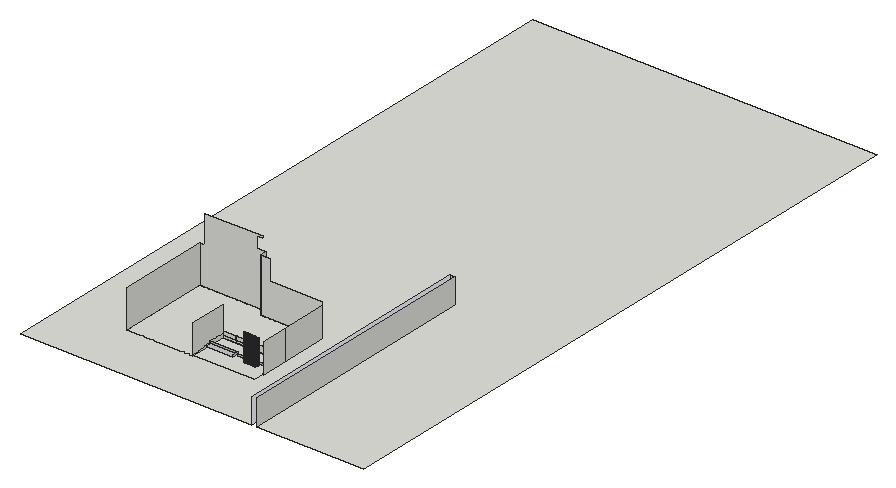
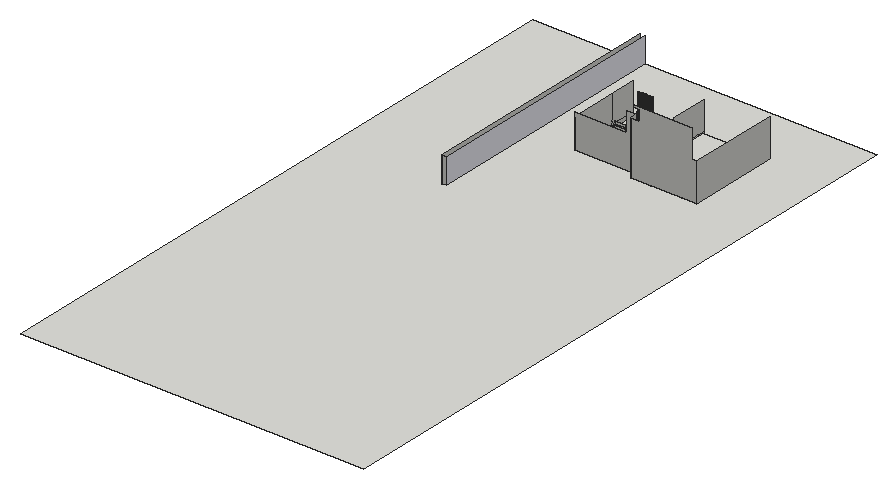
# SketchUp Ruby script. Lengths in inches.
U = 1.inch
M = Sketchup.active_model
def pt(a) = Geom::Point3d.new(a.map { |v| v * U })
def face(e, loops, mat)
  f = e.add_face(loops[0].map { |a| pt(a) })
  loops[1..].each { |l| e.add_face(l.map { |a| pt(a) }).erase! }
  f.material = f.back_material = mat if mat
  f
end
# faces: each face lists its corners as indices into pts; further lists are holes
def faces(e, pts, list, mat = nil) = list.each { |f| face(e, (f[0].is_a?(Array) ? f : [f]).map { |l| l.map { |i| pts[i] } }, mat) }
# xy, xz, yz: faces in a plane at the given z, y or x. An outline is a flat list of corners, or four numbers for a rectangle; further outlines are holes
def ring(l) = l.size == 4 ? [[l[0], l[1]], [l[2], l[1]], [l[2], l[3]], [l[0], l[3]]] : l.each_slice(2).to_a
def flat(e, list, mat, &to3) = list.each { |f| face(e, (f[0].is_a?(Array) ? f : [f]).map { |l| ring(l).map { |u, v| to3.(u, v) } }, mat) }
def xy(e, z, list, mat = nil) = flat(e, list, mat) { |x, y| [x, y, z] }
def xz(e, y, list, mat = nil) = flat(e, list, mat) { |x, z| [x, y, z] }
def yz(e, x, list, mat = nil) = flat(e, list, mat) { |y, z| [x, y, z] }
def lines(e, pts, list) = list.each { |a, b| e.add_line(pt(pts[a]), pt(pts[b])) }
# prism: a flat outline (further loops are holes) pulled along v
def prism(e, loops, v, mat = nil)
  f = face(e, loops, mat); d = Geom::Vector3d.new(v.map { |x| x * U })
  f.pushpull(f.normal.samedirection?(d) ? d.length : -d.length)
end
def box(e, o, s, mat = nil) = prism(e, [[o, [o[0] + s[0], o[1], o[2]], [o[0] + s[0], o[1] + s[1], o[2]], [o[0], o[1] + s[1], o[2]]]], [0, 0, s[2]], mat)
def at(x, y, z, deg = 0) = Geom::Transformation.translation(pt([x, y, z])) * Geom::Transformation.rotation(ORIGIN, Z_AXIS, deg.degrees)
def axes(o, x, y, z) = Geom::Transformation.new([*x, 0, *y, 0, *z, 0, *pt(o).to_a, 1])
def part(name) = M.definitions.add(name)
# library, detail: a bought-in or finely detailed component or shape, given as its bounding box
def library(name, o, s) = part(name).tap { |d| box(d.entities, o, s) }
def detail(e, o, s) = box(e.add_group.entities, o, s)
def put(e, d, t, mat = nil) = e.add_instance(d, t).tap { |i| i.material = mat if mat }
def group(e, t, mat = nil) = e.add_group.tap { |g| g.transformation = t; g.material = mat if mat }.entities
root = M.entities
M.materials.add("[0117_GhostWhite]").color = [248, 248, 255]
M.materials.add("[Polished Concrete New]").color = [200, 200, 203]
xy(root,0,[[[0,0,1769.06,0,1769.06,1887.6875,1802.44,1887.6875,1802.44,0,2622.9375,0,2622.9375,4884.1875,0,4884.1875],[465.27,433.09,465.27,1128.33,971.9,1128.33,971.9,1073.99,1443.95,1073.99,1443.95,433.09]],[465.27,433.09,971.9,433.09,971.9,719.78,1299.63,719.78,1299.63,1073.99,971.9,1073.99,971.9,1128.33,465.27,1128.33],[971.9,433.09,1443.95,433.09,1443.95,521.59,1425.51,521.59,1425.51,719.78,971.9,719.78],[1425.51,594.47,1443.95,719.78],[1299.63,719.78,1443.95,1073.99]])
xy(root,18.375,[[971.9,547.43,1182.84,594.47]],"[Polished Concrete New]")
xy(root,19.06,[[1332.64,714.35,1425.51,719.78]])
xy(root,19.16,[[971.9,714.35,1074.08,719.78],[1074.08,714.35,1176.26,719.78]])
xz(root,583.56,[[1193.75,13.1875,1414.59,29.3125]],"[Polished Concrete New]")
xz(root,594.47,[[971.9,18.375,1182.84,29.3125]],"[Polished Concrete New]")
xz(root,714.35,[[1332.64,19.06,1425.51,46.83],[971.9,19.16,1074.08,46.92],[1074.08,19.16,1176.26,46.92]])
xz(root,719.78,[[971.9,0,1074.08,19.16],[1074.08,0,1176.26,19.16],[1176.26,0,1299.63,29.3125],[1299.63,0,1332.64,29.3125],[1332.64,0,1425.51,19.06],
  [1332.64,19.06,1425.51,29.3125],[971.9,19.16,1074.08,29.3125],[1074.08,19.16,1176.26,29.3125]])
xz(root,1073.99,[[971.9,0,971.9,407.9375,1045.74,407.9375,1045.74,256.3125,1443.95,256.3125,1443.95,0]])
xz(root,1128.33,[[465.27,0,465.27,287.9375,507.79,287.9375,507.79,504.5,944.67,504.5,944.67,488.97,898.67,488.97,898.67,407.9375,971.9,407.9375,971.9,0]])
xz(root,1887.6875,[[1769.06,0,1802.44,193.9375]])
yz(root,465.27,[[433.09,0,1128.33,287.9375]])
yz(root,971.9,[[433.09,0,719.78,0,719.78,19.16,714.35,19.16,714.35,29.3125,594.47,29.3125,594.47,18.375,547.43,18.375,547.43,10.3125,490.26,10.3125,490.26,4.5,433.09,4.5],[1073.99,0,1128.33,407.9375],[[433.09,4.5,490.26,4.5,490.26,10.3125,547.43,10.3125,547.43,18.375,594.47,18.375,594.47,29.3125,714.35,29.3125,714.35,46.92,719.78,46.92,719.78,225.29,433.09,225.29],[569.58,201.42,568.92,201.51,568.3,201.76,567.77,202.17,567.36,202.7,567.1,203.32,567.02,203.98,567.1,204.64,567.36,205.26,567.77,205.79,568.3,206.2,568.92,206.46,569.58,206.54,570.24,206.46,570.86,206.2,571.39,205.79,571.8,205.26,572.05,204.64,572.14,203.98,572.05,203.32,571.8,202.7,571.39,202.17,570.86,201.76,570.24,201.51]],[714.35,19.16,719.78,29.3125]])
yz(root,1074.08,[[714.35,19.16,719.78,46.92]])
yz(root,1176.26,[[714.35,19.16,719.78,19.16,719.78,29.3125,769.53,29.3125,769.53,46.92,714.35,46.92]])
yz(root,1182.84,[[547.43,18.375,594.47,29.3125]],"[Polished Concrete New]")
yz(root,1332.64,[[714.35,19.06,719.78,46.83]])
yz(root,1425.51,[[594.47,0,594.47,29.3125,714.35,29.3125,714.35,19.06,719.78,19.06,719.78,0],[714.35,19.06,719.78,29.3125]])
yz(root,1443.95,[[521.59,0,719.78,225.29],[719.78,0,1073.99,225.29]])
yz(root,1769.06,[[0,0,1887.6875,193.9375]],"[0117_GhostWhite]")
yz(root,1802.44,[[0,0,1887.6875,193.9375]])
p = [[1253.3,565.01,0],[1253.85,564.82,0],[1253.85,564.82,202.53],[1253.3,565.01,202.53],[1254.43,564.77,0],[1254.43,564.77,202.53],
  [1255.01,564.88,0],[1255.01,564.88,202.53],[1264.05,565.01,0],[1264.6,564.82,0],[1264.6,564.82,202.53],[1264.05,565.01,202.53],
  [1265.18,564.77,0],[1265.18,564.77,202.53],[1265.76,564.88,0],[1265.76,564.88,202.53],[1274.8,565.01,0],[1275.35,564.82,0],
  [1275.35,564.82,202.53],[1274.8,565.01,202.53],[1275.93,564.77,0],[1275.93,564.77,202.53],[1276.51,564.88,0],[1276.51,564.88,202.53],
  [1285.55,565.01,0],[1286.1,564.82,0],[1286.1,564.82,202.53],[1285.55,565.01,202.53],[1286.68,564.77,0],[1286.68,564.77,202.53],
  [1287.26,564.88,0],[1287.26,564.88,202.53],[1296.3,565.01,0],[1296.85,564.82,0],[1296.85,564.82,202.53],[1296.3,565.01,202.53],
  [1297.43,564.77,0],[1297.43,564.77,202.53],[1298.01,564.88,0],[1298.01,564.88,202.53],[1307.05,565.01,0],[1307.6,564.82,0],
  [1307.6,564.82,202.53],[1307.05,565.01,202.53],[1308.18,564.77,0],[1308.18,564.77,202.53],[1308.76,564.88,0],[1308.76,564.88,202.53],
  [1317.8,565.01,0],[1318.35,564.82,0],[1318.35,564.82,202.53],[1317.8,565.01,202.53],[1318.93,564.77,0],[1318.93,564.77,202.53],
  [1319.51,564.88,0],[1319.51,564.88,202.53],[1328.55,565.01,0],[1329.1,564.82,0],[1329.1,564.82,202.53],[1328.55,565.01,202.53],
  [1329.68,564.77,0],[1329.68,564.77,202.53],[1330.26,564.88,0],[1330.26,564.88,202.53],[1339.3,565.01,0],[1339.85,564.82,0],
  [1339.85,564.82,202.53],[1339.3,565.01,202.53],[1340.43,564.77,0],[1340.43,564.77,202.53],[1341.01,564.88,0],[1341.01,564.88,202.53],
  [1255.54,565.14,0],[1255.54,565.14,202.53],[1266.29,565.14,0],[1266.29,565.14,202.53],[1277.04,565.14,0],[1277.04,565.14,202.53],
  [1287.79,565.14,0],[1287.79,565.14,202.53],[1298.54,565.14,0],[1298.54,565.14,202.53],[1309.29,565.14,0],[1309.29,565.14,202.53],
  [1320.04,565.14,0],[1320.04,565.14,202.53],[1330.79,565.14,0],[1330.79,565.14,202.53],[1341.54,565.14,0],[1341.54,565.14,202.53],
  [1252.8125,565.34,0],[1252.8125,565.34,202.53],[1263.5625,565.34,0],[1263.5625,565.34,202.53],[1274.3125,565.34,0],[1274.3125,565.34,202.53],
  [1285.0625,565.34,0],[1285.0625,565.34,202.53],[1295.8125,565.34,0],[1295.8125,565.34,202.53],[1306.5625,565.34,0],[1306.5625,565.34,202.53],
  [1317.3125,565.34,0],[1317.3125,565.34,202.53],[1328.0625,565.34,0],[1328.0625,565.34,202.53],[1338.8125,565.34,0],[1338.8125,565.34,202.53],
  [1255.98,565.52,0],[1255.98,565.52,202.53],[1266.73,565.52,0],[1266.73,565.52,202.53],[1277.48,565.52,0],[1277.48,565.52,202.53],
  [1288.23,565.52,0],[1288.23,565.52,202.53],[1298.98,565.52,0],[1298.98,565.52,202.53],[1309.73,565.52,0],[1309.73,565.52,202.53],
  [1320.48,565.52,0],[1320.48,565.52,202.53],[1331.23,565.52,0],[1331.23,565.52,202.53],[1341.98,565.52,0],[1341.98,565.52,202.53],
  [1252.43,565.78,0],[1252.43,565.78,202.53],[1263.18,565.78,0],[1263.18,565.78,202.53],[1273.93,565.78,0],[1273.93,565.78,202.53],
  [1284.68,565.78,0],[1284.68,565.78,202.53],[1295.43,565.78,0],[1295.43,565.78,202.53],[1306.18,565.78,0],[1306.18,565.78,202.53],
  [1316.93,565.78,0],[1316.93,565.78,202.53],[1327.68,565.78,0],[1327.68,565.78,202.53],[1338.43,565.78,0],[1338.43,565.78,202.53],
  [1256.3125,566.01,0],[1256.3125,566.01,202.53],[1267.0625,566.01,0],[1267.0625,566.01,202.53],[1277.8125,566.01,0],[1277.8125,566.01,202.53],
  [1288.5625,566.01,0],[1288.5625,566.01,202.53],[1299.3125,566.01,0],[1299.3125,566.01,202.53],[1310.0625,566.01,0],[1310.0625,566.01,202.53],
  [1320.8125,566.01,0],[1320.8125,566.01,202.53],[1331.5625,566.01,0],[1331.5625,566.01,202.53],[1342.3125,566.01,0],[1342.3125,566.01,202.53],
  [1252.17,566.31,0],[1252.17,566.31,202.53],[1262.92,566.31,0],[1262.92,566.31,202.53],[1273.67,566.31,0],[1273.67,566.31,202.53],
  [1284.42,566.31,0],[1284.42,566.31,202.53],[1295.17,566.31,0],[1295.17,566.31,202.53],[1305.92,566.31,0],[1305.92,566.31,202.53],
  [1316.67,566.31,0],[1316.67,566.31,202.53],[1327.42,566.31,0],[1327.42,566.31,202.53],[1338.17,566.31,0],[1338.17,566.31,202.53],
  [1256.5,566.5625,0],[1256.5,566.5625,202.53],[1267.25,566.5625,0],[1267.25,566.5625,202.53],[1278,566.5625,0],[1278,566.5625,202.53],
  [1288.75,566.5625,0],[1288.75,566.5625,202.53],[1299.5,566.5625,0],[1299.5,566.5625,202.53],[1310.25,566.5625,0],[1310.25,566.5625,202.53],
  [1321,566.5625,0],[1321,566.5625,202.53],[1331.75,566.5625,0],[1331.75,566.5625,202.53],[1342.5,566.5625,0],[1342.5,566.5625,202.53],
  [1252.0625,566.88,0],[1252.0625,566.88,202.53],[1262.8125,566.88,0],[1262.8125,566.88,202.53],[1273.5625,566.88,0],[1273.5625,566.88,202.53],
  [1284.3125,566.88,0],[1284.3125,566.88,202.53],[1295.0625,566.88,0],[1295.0625,566.88,202.53],[1305.8125,566.88,0],[1305.8125,566.88,202.53],
  [1316.5625,566.88,0],[1316.5625,566.88,202.53],[1327.3125,566.88,0],[1327.3125,566.88,202.53],[1338.0625,566.88,0],[1338.0625,566.88,202.53],
  [1256.55,567.15,0],[1256.55,567.15,202.53],[1267.3,567.15,0],[1267.3,567.15,202.53],[1278.05,567.15,0],[1278.05,567.15,202.53],
  [1288.8,567.15,0],[1288.8,567.15,202.53],[1299.55,567.15,0],[1299.55,567.15,202.53],[1310.3,567.15,0],[1310.3,567.15,202.53],
  [1321.05,567.15,0],[1321.05,567.15,202.53],[1331.8,567.15,0],[1331.8,567.15,202.53],[1342.55,567.15,0],[1342.55,567.15,202.53],
  [1252.1,567.47,0],[1252.1,567.47,202.53],[1262.85,567.47,0],[1262.85,567.47,202.53],[1273.6,567.47,0],[1273.6,567.47,202.53],
  [1284.35,567.47,0],[1284.35,567.47,202.53],[1295.1,567.47,0],[1295.1,567.47,202.53],[1305.85,567.47,0],[1305.85,567.47,202.53],
  [1316.6,567.47,0],[1316.6,567.47,202.53],[1327.35,567.47,0],[1327.35,567.47,202.53],[1338.1,567.47,0],[1338.1,567.47,202.53],
  [1256.44,567.72,0],[1256.44,567.72,202.53],[1267.19,567.72,0],[1267.19,567.72,202.53],[1277.94,567.72,0],[1277.94,567.72,202.53],
  [1288.69,567.72,0],[1288.69,567.72,202.53],[1299.44,567.72,0],[1299.44,567.72,202.53],[1310.19,567.72,0],[1310.19,567.72,202.53],
  [1320.94,567.72,0],[1320.94,567.72,202.53],[1331.69,567.72,0],[1331.69,567.72,202.53],[1342.44,567.72,0],[1342.44,567.72,202.53],
  [1252.3,568.02,0],[1252.3,568.02,202.53],[1263.05,568.02,0],[1263.05,568.02,202.53],[1273.8,568.02,0],[1273.8,568.02,202.53],
  [1284.55,568.02,0],[1284.55,568.02,202.53],[1295.3,568.02,0],[1295.3,568.02,202.53],[1306.05,568.02,0],[1306.05,568.02,202.53],
  [1316.8,568.02,0],[1316.8,568.02,202.53],[1327.55,568.02,0],[1327.55,568.02,202.53],[1338.3,568.02,0],[1338.3,568.02,202.53],
  [1256.18,568.25,0],[1256.18,568.25,202.53],[1266.93,568.25,0],[1266.93,568.25,202.53],[1277.68,568.25,0],[1277.68,568.25,202.53],
  [1288.43,568.25,0],[1288.43,568.25,202.53],[1299.18,568.25,0],[1299.18,568.25,202.53],[1309.93,568.25,0],[1309.93,568.25,202.53],
  [1320.68,568.25,0],[1320.68,568.25,202.53],[1331.43,568.25,0],[1331.43,568.25,202.53],[1342.18,568.25,0],[1342.18,568.25,202.53],
  [1252.625,568.51,0],[1252.625,568.51,202.53],[1263.375,568.51,0],[1263.375,568.51,202.53],[1274.125,568.51,0],[1274.125,568.51,202.53],
  [1284.875,568.51,0],[1284.875,568.51,202.53],[1295.625,568.51,0],[1295.625,568.51,202.53],[1306.375,568.51,0],[1306.375,568.51,202.53],
  [1317.125,568.51,0],[1317.125,568.51,202.53],[1327.875,568.51,0],[1327.875,568.51,202.53],[1338.625,568.51,0],[1338.625,568.51,202.53],
  [1255.8,568.69,0],[1255.8,568.69,202.53],[1266.55,568.69,0],[1266.55,568.69,202.53],[1277.3,568.69,0],[1277.3,568.69,202.53],
  [1288.05,568.69,0],[1288.05,568.69,202.53],[1298.8,568.69,0],[1298.8,568.69,202.53],[1309.55,568.69,0],[1309.55,568.69,202.53],
  [1320.3,568.69,0],[1320.3,568.69,202.53],[1331.05,568.69,0],[1331.05,568.69,202.53],[1341.8,568.69,0],[1341.8,568.69,202.53],
  [1253.07,568.89,0],[1253.07,568.89,202.53],[1263.82,568.89,0],[1263.82,568.89,202.53],[1274.57,568.89,0],[1274.57,568.89,202.53],
  [1285.32,568.89,0],[1285.32,568.89,202.53],[1296.07,568.89,0],[1296.07,568.89,202.53],[1306.82,568.89,0],[1306.82,568.89,202.53],
  [1317.57,568.89,0],[1317.57,568.89,202.53],[1328.32,568.89,0],[1328.32,568.89,202.53],[1339.07,568.89,0],[1339.07,568.89,202.53],
  [1255.3125,569.02,0],[1255.3125,569.02,202.53],[1266.0625,569.02,0],[1266.0625,569.02,202.53],[1276.8125,569.02,0],[1276.8125,569.02,202.53],
  [1287.5625,569.02,0],[1287.5625,569.02,202.53],[1298.3125,569.02,0],[1298.3125,569.02,202.53],[1309.0625,569.02,0],[1309.0625,569.02,202.53],
  [1319.8125,569.02,0],[1319.8125,569.02,202.53],[1330.5625,569.02,0],[1330.5625,569.02,202.53],[1341.3125,569.02,0],[1341.3125,569.02,202.53],
  [1253.6,569.15,0],[1253.6,569.15,202.53],[1264.35,569.15,0],[1264.35,569.15,202.53],[1275.1,569.15,0],[1275.1,569.15,202.53],
  [1285.85,569.15,0],[1285.85,569.15,202.53],[1296.6,569.15,0],[1296.6,569.15,202.53],[1307.35,569.15,0],[1307.35,569.15,202.53],
  [1318.1,569.15,0],[1318.1,569.15,202.53],[1328.85,569.15,0],[1328.85,569.15,202.53],[1339.6,569.15,0],[1339.6,569.15,202.53],
  [1254.76,569.22,0],[1254.76,569.22,202.53],[1265.51,569.22,0],[1265.51,569.22,202.53],[1276.26,569.22,0],[1276.26,569.22,202.53],
  [1287.01,569.22,0],[1287.01,569.22,202.53],[1297.76,569.22,0],[1297.76,569.22,202.53],[1308.51,569.22,0],[1308.51,569.22,202.53],
  [1319.26,569.22,0],[1319.26,569.22,202.53],[1330.01,569.22,0],[1330.01,569.22,202.53],[1340.76,569.22,0],[1340.76,569.22,202.53],
  [1254.17,569.26,0],[1254.17,569.26,202.53],[1264.92,569.26,0],[1264.92,569.26,202.53],[1275.67,569.26,0],[1275.67,569.26,202.53],
  [1286.42,569.26,0],[1286.42,569.26,202.53],[1297.17,569.26,0],[1297.17,569.26,202.53],[1307.92,569.26,0],[1307.92,569.26,202.53],
  [1318.67,569.26,0],[1318.67,569.26,202.53],[1329.42,569.26,0],[1329.42,569.26,202.53],[1340.17,569.26,0],[1340.17,569.26,202.53],
  [1332.64,719.78,46.92],[1176.26,714.35,46.92],[1176.26,714.35,19.16],[1176.26,714.35,0],[1332.64,719.78,0],[1332.64,719.78,19.06],
  [1332.64,719.78,29.3125],[1332.64,719.78,46.83],[1359.6,567.47,202.53],[1359.6,567.47,13.1875],[1359.5625,566.88,13.1875],[1359.5625,566.88,202.53],
  [1364.05,567.15,202.53],[1364.05,567.15,13.1875],[1363.94,567.72,13.1875],[1363.94,567.72,202.53],[1359.8,568.02,202.53],[1359.8,568.02,13.1875],
  [1363.68,568.25,13.1875],[1363.68,568.25,202.53],[1360.125,568.51,202.53],[1360.125,568.51,13.1875],[1363.3,568.69,13.1875],[1363.3,568.69,202.53],
  [1360.57,568.89,202.53],[1360.57,568.89,13.1875],[1362.8125,569.02,13.1875],[1362.8125,569.02,202.53],[1361.1,569.15,202.53],[1361.1,569.15,13.1875],
  [1362.26,569.22,13.1875],[1362.26,569.22,202.53],[1361.67,569.26,202.53],[1361.67,569.26,13.1875]]
faces(root,p,[[0,1,2,3],[1,4,5,2],[4,6,7,5],[8,9,10,11],[9,12,13,10],[12,14,15,13],[16,17,18,19],[17,20,21,18],
  [20,22,23,21],[24,25,26,27],[25,28,29,26],[28,30,31,29],[32,33,34,35],[33,36,37,34],[36,38,39,37],[40,41,42,43],
  [41,44,45,42],[44,46,47,45],[48,49,50,51],[49,52,53,50],[52,54,55,53],[56,57,58,59],[57,60,61,58],[60,62,63,61],
  [64,65,66,67],[65,68,69,66],[68,70,71,69],[6,72,73,7],[14,74,75,15],[22,76,77,23],[30,78,79,31],[38,80,81,39],
  [46,82,83,47],[54,84,85,55],[62,86,87,63],[70,88,89,71],[90,0,3,91],[92,8,11,93],[94,16,19,95],[96,24,27,97],
  [98,32,35,99],[100,40,43,101],[102,48,51,103],[104,56,59,105],[106,64,67,107],[72,108,109,73],[74,110,111,75],[76,112,113,77],
  [78,114,115,79],[80,116,117,81],[82,118,119,83],[84,120,121,85],[86,122,123,87],[88,124,125,89],[126,90,91,127],[128,92,93,129],
  [130,94,95,131],[132,96,97,133],[134,98,99,135],[136,100,101,137],[138,102,103,139],[140,104,105,141],[142,106,107,143],[108,144,145,109],
  [110,146,147,111],[112,148,149,113],[114,150,151,115],[116,152,153,117],[118,154,155,119],[120,156,157,121],[122,158,159,123],[124,160,161,125],
  [162,126,127,163],[164,128,129,165],[166,130,131,167],[168,132,133,169],[170,134,135,171],[172,136,137,173],[174,138,139,175],[176,140,141,177],
  [178,142,143,179],[144,180,181,145],[146,182,183,147],[148,184,185,149],[150,186,187,151],[152,188,189,153],[154,190,191,155],[156,192,193,157],
  [158,194,195,159],[160,196,197,161],[198,162,163,199],[200,164,165,201],[202,166,167,203],[204,168,169,205],[206,170,171,207],[208,172,173,209],
  [210,174,175,211],[212,176,177,213],[214,178,179,215],[180,216,217,181],[182,218,219,183],[184,220,221,185],[186,222,223,187],[188,224,225,189],
  [190,226,227,191],[192,228,229,193],[194,230,231,195],[196,232,233,197],[234,198,199,235],[236,200,201,237],[238,202,203,239],[240,204,205,241],
  [242,206,207,243],[244,208,209,245],[246,210,211,247],[248,212,213,249],[250,214,215,251],[216,252,253,217],[218,254,255,219],[220,256,257,221],
  [222,258,259,223],[224,260,261,225],[226,262,263,227],[228,264,265,229],[230,266,267,231],[232,268,269,233],[270,234,235,271],[272,236,237,273],
  [274,238,239,275],[276,240,241,277],[278,242,243,279],[280,244,245,281],[282,246,247,283],[284,248,249,285],[286,250,251,287],[252,288,289,253],
  [254,290,291,255],[256,292,293,257],[258,294,295,259],[260,296,297,261],[262,298,299,263],[264,300,301,265],[266,302,303,267],[268,304,305,269],
  [306,270,271,307],[308,272,273,309],[310,274,275,311],[312,276,277,313],[314,278,279,315],[316,280,281,317],[318,282,283,319],[320,284,285,321],
  [322,286,287,323],[288,324,325,289],[290,326,327,291],[292,328,329,293],[294,330,331,295],[296,332,333,297],[298,334,335,299],[300,336,337,301],
  [302,338,339,303],[304,340,341,305],[342,306,307,343],[344,308,309,345],[346,310,311,347],[348,312,313,349],[350,314,315,351],[352,316,317,353],
  [354,318,319,355],[356,320,321,357],[358,322,323,359],[324,360,361,325],[326,362,363,327],[328,364,365,329],[330,366,367,331],[332,368,369,333],
  [334,370,371,335],[336,372,373,337],[338,374,375,339],[340,376,377,341],[378,342,343,379],[380,344,345,381],[382,346,347,383],[384,348,349,385],
  [386,350,351,387],[388,352,353,389],[390,354,355,391],[392,356,357,393],[394,358,359,395],[360,396,397,361],[362,398,399,363],[364,400,401,365],
  [366,402,403,367],[368,404,405,369],[370,406,407,371],[372,408,409,373],[374,410,411,375],[376,412,413,377],[414,378,379,415],[416,380,381,417],
  [418,382,383,419],[420,384,385,421],[422,386,387,423],[424,388,389,425],[426,390,391,427],[428,392,393,429],[430,394,395,431],[396,414,415,397],
  [398,416,417,399],[400,418,419,401],[402,420,421,403],[404,422,423,405],[406,424,425,407],[408,426,427,409],[410,428,429,411],[412,430,431,413],
  [432,433,434,435,436,437,438,439],[440,441,442,443],[444,445,446,447],[448,449,441,440],[447,446,450,451],[452,453,449,448],[451,450,454,455],[456,457,453,452],
  [455,454,458,459],[460,461,457,456],[459,458,462,463],[464,465,461,460],[463,462,465,464]])
